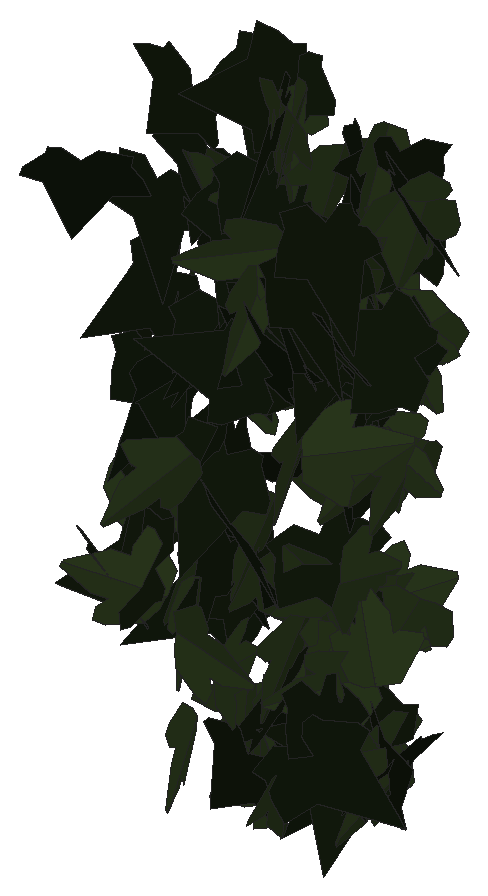
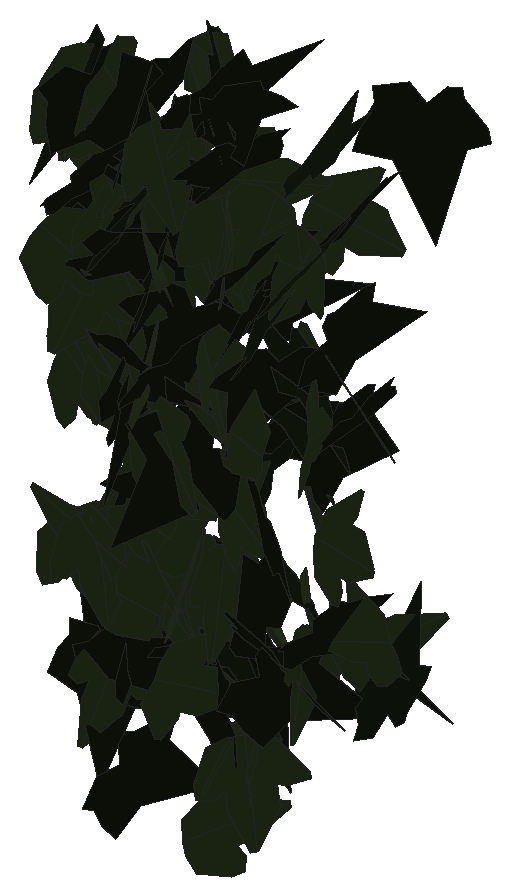
# SketchUp Ruby script. Lengths in inches.
U = 1.inch
M = Sketchup.active_model
def pt(a) = Geom::Point3d.new(a.map { |v| v * U })
def face(e, loops, mat)
  f = e.add_face(loops[0].map { |a| pt(a) })
  loops[1..].each { |l| e.add_face(l.map { |a| pt(a) }).erase! }
  f.material = f.back_material = mat if mat
  f
end
# faces: each face lists its corners as indices into pts; further lists are holes
def faces(e, pts, list, mat = nil) = list.each { |f| face(e, (f[0].is_a?(Array) ? f : [f]).map { |l| l.map { |i| pts[i] } }, mat) }
# xy, xz, yz: faces in a plane at the given z, y or x. An outline is a flat list of corners, or four numbers for a rectangle; further outlines are holes
def ring(l) = l.size == 4 ? [[l[0], l[1]], [l[2], l[1]], [l[2], l[3]], [l[0], l[3]]] : l.each_slice(2).to_a
def flat(e, list, mat, &to3) = list.each { |f| face(e, (f[0].is_a?(Array) ? f : [f]).map { |l| ring(l).map { |u, v| to3.(u, v) } }, mat) }
def xy(e, z, list, mat = nil) = flat(e, list, mat) { |x, y| [x, y, z] }
def xz(e, y, list, mat = nil) = flat(e, list, mat) { |x, z| [x, y, z] }
def yz(e, x, list, mat = nil) = flat(e, list, mat) { |y, z| [x, y, z] }
def lines(e, pts, list) = list.each { |a, b| e.add_line(pt(pts[a]), pt(pts[b])) }
# prism: a flat outline (further loops are holes) pulled along v
def prism(e, loops, v, mat = nil)
  f = face(e, loops, mat); d = Geom::Vector3d.new(v.map { |x| x * U })
  f.pushpull(f.normal.samedirection?(d) ? d.length : -d.length)
end
def box(e, o, s, mat = nil) = prism(e, [[o, [o[0] + s[0], o[1], o[2]], [o[0] + s[0], o[1] + s[1], o[2]], [o[0], o[1] + s[1], o[2]]]], [0, 0, s[2]], mat)
def at(x, y, z, deg = 0) = Geom::Transformation.translation(pt([x, y, z])) * Geom::Transformation.rotation(ORIGIN, Z_AXIS, deg.degrees)
def axes(o, x, y, z) = Geom::Transformation.new([*x, 0, *y, 0, *z, 0, *pt(o).to_a, 1])
def part(name) = M.definitions.add(name)
# library, detail: a bought-in or finely detailed component or shape, given as its bounding box
def library(name, o, s) = part(name).tap { |d| box(d.entities, o, s) }
def detail(e, o, s) = box(e.add_group.entities, o, s)
def put(e, d, t, mat = nil) = e.add_instance(d, t).tap { |i| i.material = mat if mat }
def group(e, t, mat = nil) = e.add_group.tap { |g| g.transformation = t; g.material = mat if mat }.entities
root = M.entities
M.materials.add("efeu1").color = [18, 25, 13]
M.materials.add("efeu2").color = [43, 57, 29]
c1 = part("ivyleaf_10")
p = [[0,0.5,-0.03],[-0.0625,2.02,-0.43],[-0.19,2.01,-0.46],[-0.54,1.05,-0.29],[-0.52,0.625,-0.18],[-0.83,0.76,-0.28],
  [-1.16,0.64,-0.33],[-1.15,0.33,-0.24],[-0.77,-0.39,0.02],[-0.3,-0.51,0.16],[0.04,-0.48,0.23],[-0.02,2.01,-0.4375],
  [-0.06,2.01,-0.43],[0.04,-0.49,0.23],[0.67,-0.49,0.14],[1.38,0.36,-0.2],[1.375,0.51,-0.24],[0.81,0.65,-0.19],
  [0.62,0.59,-0.15],[0.6,1.09,-0.28],[0.5,1.23,-0.31]]
faces(c1.entities,p,[[0,1,2,3,4,5,6,7,8,9,10],[11,12,0,13,14,15,16,17,18,19,20]],"efeu2")
c2 = part("ivyleaf_9")
p = [[1.54,2.16,1.25],[1.36,2.04,1.19],[-0.21,0.99,0.68],[-0.71,1.11,0.82],[-0.85,0.86,0.67],[-0.8,0.17,0.21],
  [-0.9,-0.01,0.1],[-0.67,-0.16,-0.02],[-0.08,-0.08,-0.05],[-0.03,-0.6,-0.4],[0.65,-0.88,-0.66],[0.83,-0.6,-0.49],
  [1.29,-0.42,-0.43],[1.8125,-0.07,-0.26],[1.21,0.44,0.15]]
faces(c2.entities,p,[[0,1,2,3,4,5,6,7,8,9,10,11,12,13,14]],"efeu1")
put(root,c1,axes([28.7,219.16,219.66],[-0.09561,-0.27341,0.40756],[-0.13235,-0.38548,-0.28964],[0.47259,-0.16326,0.00134]))
put(root,c1,axes([28.93,219.18,217.42],[0.02177,-0.04563,0.49744],[0.49761,0.04558,-0.0176],[-0.04374,0.49582,0.0474]))
put(root,c1,axes([28.72,219.39,216.11],[0.3565,-0.35058,0.0014],[0.00435,0.00243,-0.49998],[0.35056,0.35649,0.00478]))
put(root,c2,axes([26.43,220.35,222.25],[0.2485,0.34039,-0.26904],[-0.16173,-0.21502,-0.42144],[-0.40261,0.29647,0.00324]))
put(root,c2,axes([29.17,220.77,221.54],[0.23996,-0.43001,-0.08665],[-0.03517,0.07959,-0.49237],[0.43725,0.24239,0.00795]))
put(root,c1,axes([29.01,220.82,215.05],[0.04129,-0.48554,-0.11203],[-0.01025,0.11156,-0.48729],[0.49819,0.04254,-0.00074]))
put(root,c2,axes([29.35,220.74,215.52],[0.01382,-0.12857,-0.48299],[0.15949,0.45905,-0.11763],[0.47368,-0.15081,0.0537]))
put(root,c2,axes([29.38,221.08,222.13],[0.04971,-0.47286,-0.1547],[-0.01352,0.15413,-0.47546],[0.49734,0.05145,0.00254]))
put(root,c2,axes([28.66,221.33,220.48],[0.02304,-0.23508,0.44069],[0.13766,-0.42108,-0.23182],[0.48013,0.13201,0.04531]))
put(root,c2,axes([28.35,220.93,215.03],[0.19797,0.07499,-0.45297],[-0.42906,-0.14538,-0.21159],[-0.16344,0.47248,0.00678]))
put(root,c1,axes([27.83,221.22,215.79],[0.18255,-0.28336,-0.3693],[0.27504,-0.25438,0.33113],[-0.37554,-0.32404,0.06299]))
put(root,c2,axes([27.83,221.27,217.75],[0.22176,-0.3354,0.2972],[0.17485,-0.24055,-0.40195],[0.41261,0.2822,0.0106]))
put(root,c2,axes([27.67,221.39,218.41],[-0.23348,-0.44123,0.02835],[-0.00856,-0.02755,-0.49917],[0.44205,-0.23358,0.00531]))
put(root,c1,axes([28.17,221.4,220.74],[0.06742,0.364,-0.33609],[-0.06695,-0.32938,-0.37017],[-0.49089,0.09491,0.00433]))
put(root,c2,axes([28.18,221.36,219.68],[-0.17671,0.00384,0.46772],[-0.46563,-0.0488,-0.17552],[0.0443,-0.4976,0.02083]))
put(root,c2,axes([29.03,221.43,220.44],[0.45581,-0.17616,-0.10584],[0.10647,-0.01782,0.48821],[-0.17578,-0.4676,0.02127]))
put(root,c2,axes([29.17,221.25,215.87],[0.17957,-0.43225,-0.17583],[-0.06591,0.16301,-0.46806],[0.46196,0.19128,0.00157]))
put(root,c1,axes([28.21,221.42,221.27],[0.00952,0.09572,-0.49066],[-0.44233,-0.22704,-0.05288],[-0.23292,0.43508,0.08035]))
put(root,c2,axes([28.03,221.4375,219.92],[0.13566,-0.14789,0.45796],[0.33744,-0.31001,-0.20007],[0.34312,0.36335,0.0157]))
put(root,c1,axes([27.07,221.52,216.34],[0.35206,-0.26696,0.23406],[0.1784,-0.15198,-0.44167],[0.30696,0.39451,-0.01176]))
put(root,c2,axes([26.49,221.63,221.45],[0.0668,-0.48608,0.09622],[0.02669,-0.09342,-0.49047],[0.4948,0.07067,0.01347]))
put(root,c2,axes([28.91,221.73,220.37],[-0.0675,-0.4709,0.15395],[-0.03557,-0.15036,-0.47553],[0.49415,-0.07514,-0.0132]))
put(root,c1,axes([29.3125,221.13,219.2],[0.04861,-0.05735,-0.49432],[0.39585,0.30543,0.00349],[0.30156,-0.39169,0.07509]))
put(root,c1,axes([26.29,221.66,216.14],[0.11234,0.20323,0.44281],[-0.20859,-0.39061,0.23219],[0.44031,-0.2369,-0.00298]))
put(root,c1,axes([28.43,221.67,216.26],[0.0828,-0.41923,0.2596],[0.08923,-0.24615,-0.42597],[0.48496,0.11687,0.03406]))
put(root,c2,axes([28.5,221.39,215.68],[-0.35036,0.35599,-0.02271],[0.01212,-0.01993,-0.49946],[-0.35651,-0.35053,0.00533]))
put(root,c1,axes([28.51,221.6875,218.87],[0.15182,-0.39422,0.26747],[0.13558,-0.23336,-0.4209],[0.45669,0.20033,0.03604]))
put(root,c2,axes([26.49,221.86,218.84],[0.00288,-0.01146,-0.49986],[0.29005,-0.40712,0.011],[-0.40726,-0.29004,0.00431]))
put(root,c2,axes([29.19,221.73,215.0625],[-0.24371,-0.42591,-0.09596],[0.05035,0.08174,-0.4907],[0.43367,-0.24884,0.00305]))
put(root,c1,axes([29.64,221.91,214.77],[0.05305,-0.21525,0.44817],[0.0847,-0.44021,-0.22145],[0.48991,0.09942,-0.01025]))
put(root,c2,axes([26.45,221.96,220.11],[0.03464,-0.19944,-0.45719],[0.17323,-0.42496,0.1985],[-0.46775,-0.17215,0.03966]))
put(root,c2,axes([29.99,221.8,220.375],[-0.19617,-0.38502,-0.25155],[-0.10744,-0.22754,0.43207],[-0.44718,0.22357,0.00654]))
put(root,c1,axes([29.1875,221.76,215.9],[0.10859,0.12482,-0.47183],[-0.42786,-0.20822,-0.15355],[-0.23482,0.43711,0.06159]))
put(root,c2,axes([27.6,221.47,218.83],[-0.29344,0.3813,0.13603],[-0.09638,0.09738,-0.48086],[-0.3932,-0.30843,0.01635]))
put(root,c1,axes([27.83,221.89,217.54],[0.09572,-0.39286,0.29411],[0.11191,-0.27428,-0.4028],[0.47782,0.14294,0.03543]))
put(root,c2,axes([27.55,221.35,216.66],[-0.36639,0.1511,-0.30484],[-0.28153,0.11692,0.39632],[0.19105,0.46206,-0.0006]))
put(root,c2,axes([26.3125,221.78,219.11],[0.13386,-0.47422,-0.08485],[-0.02656,0.08067,-0.49273],[0.48102,0.13642,-0.00359]))
put(root,c2,axes([28.12,221.85,222.93],[-0.32825,0.1441,-0.34855],[0.31496,-0.14948,-0.35841],[-0.2075,-0.45485,0.00736]))
put(root,c2,axes([27.7,222.12,219.73],[-0.05327,-0.274,0.41483],[-0.05708,-0.41108,-0.27885],[0.49387,-0.07707,0.01252]))
put(root,c2,axes([29.49,221.95,214.75],[0.00895,-0.0143,0.49972],[0.21171,-0.45266,-0.01674],[0.45288,0.21189,-0.00205]))
put(root,c2,axes([25.64,221.99,215.875],[0.39691,-0.29632,-0.06822],[0.06323,-0.02929,0.49512],[-0.29742,-0.40167,0.01422]))
put(root,c1,axes([28.77,221.97,216.83],[-0.32371,-0.2417,-0.29461],[-0.18714,-0.2359,0.39916],[-0.33196,0.36869,0.06226]))
put(root,c2,axes([27.24,221.65,219.57],[-0.30711,0.39418,-0.01749],[0.00713,-0.01661,-0.49967],[-0.3945,-0.30716,0.00458]))
put(root,c1,axes([29.4375,222.05,218.77],[-0.06073,-0.28881,0.40361],[-0.06338,-0.39877,-0.29489],[0.49223,-0.08698,0.01183]))
put(root,c2,axes([26.34,221.72,216.39],[-0.4031,0.19572,0.22183],[-0.20034,0.09527,-0.44809],[-0.21766,-0.45013,0.00162]))
put(root,c1,axes([29.58,221.68,216.33],[0.46188,0.08604,0.17106],[-0.1747,0.00652,0.46844],[0.07838,-0.4925,0.03608]))
put(root,c2,axes([29.43,222.04,215],[-0.16198,-0.0601,0.4692],[-0.44629,-0.14498,-0.17264],[0.1568,-0.47473,-0.00667]))
put(root,c1,axes([28.48,222.02,215.85],[-0.02745,-0.02721,-0.4985],[0.34193,-0.3648,0.00108],[-0.36377,-0.34085,0.03864]))
put(root,c2,axes([28.875,222.1,221.06],[-0.06918,-0.49248,0.05179],[-0.00655,-0.05138,-0.49731],[0.49515,-0.06949,0.00066]))
put(root,c1,axes([29.37,221.51,217.42],[0.00592,-0.16458,-0.4721],[0.08451,0.46567,-0.16128],[0.49277,-0.07789,0.03333]))
put(root,c1,axes([28.23,221.76,222.89],[-0.41938,0.17149,0.21145],[-0.21268,0.03606,-0.45107],[-0.16996,-0.46829,0.0427]))
put(root,c2,axes([28.71,221.85,217.54],[-0.00447,-0.33806,-0.36837],[0.1627,0.34735,-0.32075],[0.47277,-0.12274,0.1069]))
put(root,c2,axes([26.45,222.29,222.35],[-0.16905,-0.27839,0.37937],[0.0698,-0.41348,-0.27232],[0.46535,-0.03911,0.17866]))
put(root,c1,axes([29.08,222.08,221.03],[-0.27917,0.04649,0.41219],[0.38525,-0.15513,0.27842],[0.15377,0.47305,0.0508]))
put(root,c2,axes([27.78,221.93,221.96],[0.09967,-0.41651,-0.25805],[0.04083,0.26948,-0.41918],[0.48826,0.06249,0.08773]))
put(root,c2,axes([29.09,222.34,218.49],[-0.03945,-0.06495,0.49419],[-0.20888,-0.44795,-0.07555],[0.45256,-0.21241,0.00821]))
put(root,c2,axes([27.1875,222.2,216.48],[0.10771,-0.1414,0.46734],[0.26087,-0.38787,-0.17748],[0.41273,0.28207,-0.00978]))
put(root,c2,axes([29.72,221.7,214.94],[-0.00003,0.49366,0.0794],[0.00006,0.0794,-0.49366],[-0.5,-0.00002,-0.00006]))
put(root,c2,axes([29.28,222,220.88],[-0.42094,-0.16819,-0.21099],[-0.19552,-0.07932,0.4533],[-0.18595,0.46413,0.001]))
put(root,c1,axes([29.72,222.24,218.78],[-0.05701,-0.43012,0.24848],[-0.03046,-0.24662,-0.43388],[0.4958,-0.06461,0.00192]))
put(root,c2,axes([27.73,222.2,215.18],[0.08788,-0.09066,-0.4838],[0.49222,0.01582,0.08644],[-0.00037,-0.49146,0.09203]))
put(root,c1,axes([29.91,222.12,222.02],[-0.2324,-0.42962,0.10682],[-0.05008,-0.09436,-0.48846],[0.43986,-0.23774,0.00083]))
put(root,c1,axes([28.12,222.125,222.79],[0.29529,-0.402,0.03463],[0.02031,-0.02806,-0.4988],[0.40298,0.29599,-0.00024]))
put(root,c1,axes([27.35,222.25,214.61],[-0.06215,-0.03309,0.49502],[0.44692,-0.22034,0.04138],[0.21541,0.44761,0.05697]))
put(root,c2,axes([27.72,222.4,222.71],[-0.16142,-0.08671,0.46522],[-0.30485,-0.3569,-0.1723],[0.36195,-0.33927,0.06235]))
put(root,c1,axes([29.8125,221.94,222.27],[-0.23008,-0.41036,-0.16932],[0.08377,0.14715,-0.47046],[0.43594,-0.24485,0.00104]))
put(root,c2,axes([29.6,222.13,219.93],[0.00117,0.0296,0.49912],[-0.48931,0.10272,-0.00494],[-0.10284,-0.48844,0.02921]))
put(root,c1,axes([27.61,222.11,214.875],[-0.0839,0.47089,-0.14568],[0.02037,-0.14434,-0.47828],[-0.49249,-0.08619,0.00503]))
put(root,c1,axes([29.36,222.42,220.54],[-0.0501,0.13372,0.47918],[0.03554,-0.47941,0.1375],[0.49621,0.04784,0.03853]))
put(root,c2,axes([25.94,222.3,219.81],[-0.34755,-0.06335,-0.35383],[0.35917,-0.08112,-0.33826],[-0.01455,-0.48929,0.10189]))
put(root,c1,axes([29.43,222.25,218.79],[-0.0869,-0.05418,-0.4894],[0.41658,-0.27304,-0.04374],[-0.26251,-0.41535,0.0926]))
put(root,c2,axes([28.55,222.41,220.37],[0.23218,-0.18571,-0.402],[0.36373,-0.17892,0.29273],[-0.25258,-0.42837,0.05201]))
put(root,c1,axes([29.42,221.92,215.14],[-0.18699,-0.38251,-0.26215],[0.1,0.24275,-0.42553],[0.45281,-0.21157,-0.01428]))
put(root,c1,axes([29.31,222.06,221.81],[-0.29787,-0.38985,-0.09641],[0.05484,0.07942,-0.4906],[0.39783,-0.30284,-0.00456]))
put(root,c1,axes([27.84,222.05,216.85],[-0.07123,-0.46881,-0.15856],[0.04694,0.15307,-0.47367],[0.49267,-0.08237,0.02221]))
put(root,c2,axes([28.34,222.03,219.84],[-0.04685,-0.23935,-0.43648],[0.1648,0.40623,-0.24045],[0.46973,-0.16639,0.04082]))
put(root,c2,axes([27.19,222.46,220.99],[-0.11546,-0.47738,0.09368],[-0.00818,-0.09436,-0.49095],[0.48642,-0.1149,0.01398]))
put(root,c1,axes([28.64,222.3,220.81],[0.23225,-0.42777,0.11434],[0.05386,-0.10086,-0.48675],[0.4395,0.23841,-0.00077]))
put(root,c1,axes([27.73,222.5,213.79],[0.00324,0.08649,0.49245],[-0.0841,-0.48535,0.08579],[0.49287,-0.08338,0.0114]))
put(root,c1,axes([27.48,222.45,221.11],[-0.09185,0.19167,-0.45258],[0.124,-0.43648,-0.21002],[-0.47559,-0.15082,0.03265]))
put(root,c1,axes([29.23,222.34,222.58],[-0.00142,0.41474,-0.27926],[-0.06058,-0.27735,-0.41159],[-0.49631,0.03267,0.05104]))
put(root,c1,axes([27.93,222.25,222.63],[-0.04796,0.47854,-0.13674],[0.01536,-0.13588,-0.48094],[-0.49746,-0.05034,-0.00167]))
put(root,c2,axes([29.625,222.1,222.37],[0.41683,-0.16053,-0.22468],[-0.20517,0.09223,-0.44654],[0.18481,0.46446,0.01101]))
put(root,c1,axes([29.66,222.3,216.76],[-0.36128,-0.26089,0.22674],[-0.18665,-0.1288,-0.44561],[0.29092,-0.40663,-0.00433]))
put(root,c2,axes([26.9,222.54,216.04],[-0.02314,-0.04708,-0.49724],[-0.08554,-0.49005,0.05038],[-0.49209,0.0874,0.01462]))
put(root,c2,axes([28.9,222.41,220.99],[0.25051,-0.41543,0.12109],[0.06616,-0.10151,-0.4851],[0.42763,0.25907,0.00411]))
put(root,c2,axes([29.0625,221.99,218.73],[0.13186,-0.11039,-0.4695],[-0.37795,0.27871,-0.17168],[0.29961,0.40017,-0.00995]))
put(root,c1,axes([27.82,222.39,220.75],[-0.22267,0.00437,0.44766],[0.43208,-0.12874,0.21618],[0.11716,0.48312,0.05355]))
put(root,c2,axes([26.88,222.54,220.36],[0.13536,-0.42557,0.22487],[0.04983,-0.21994,-0.44625],[0.47874,0.14322,-0.01713]))
put(root,c1,axes([28.34,222.2,216.26],[-0.20267,0.45533,-0.03998],[-0.03745,0.02704,0.49786],[0.45555,0.20479,0.02315]))
put(root,c2,axes([28.7,222.6,222.14],[0.16962,-0.13236,-0.45134],[0.39625,-0.21828,0.21293],[-0.2534,-0.42993,0.03085]))
put(root,c1,axes([26.62,222.16,216.33],[0.05023,-0.43839,-0.23514],[0.01717,0.23772,-0.43954],[0.49717,0.03608,0.03893]))
put(root,c2,axes([29.14,222.58,220.49],[-0.39903,-0.18804,0.2354],[-0.20175,-0.12339,-0.44054],[0.22377,-0.44656,0.0226]))
put(root,c2,axes([26.96,222.25,219.75],[-0.03191,-0.36688,-0.3382],[0.02703,0.33713,-0.36826],[0.49825,-0.04179,-0.00168]))
put(root,c1,axes([28.84,222.23,216.14],[-0.13773,-0.0462,0.47843],[0.44666,0.17154,0.14515],[-0.17755,0.46737,-0.00598]))
put(root,c1,axes([27.13,222.25,221.55],[-0.48969,0.06706,-0.07553],[0.07487,-0.00998,-0.49426],[-0.0678,-0.49538,-0.00027]))
put(root,c2,axes([29.36,222.4,222.49],[-0.01131,0.31651,-0.3869],[-0.01923,-0.38699,-0.31602],[-0.4995,0.00773,0.02093]))
put(root,c1,axes([29.35,222.36,216.89],[-0.29545,-0.4002,0.05047],[-0.02685,-0.0429,-0.49743],[0.40248,-0.29664,0.00386]))
put(root,c1,axes([27.61,222.36,221.35],[-0.36496,-0.31961,0.12105],[-0.09451,-0.07581,-0.4851],[0.32844,-0.37697,-0.00508]))
put(root,c1,axes([29.21,222.33,219.8],[-0.45007,-0.09969,0.19364],[-0.18111,-0.07562,-0.45987],[0.12097,-0.48409,0.03196]))
put(root,c2,axes([26.94,222.48,217.96],[-0.24999,0.01679,-0.43269],[0.43096,-0.03904,-0.25051],[-0.0422,-0.49819,0.00505]))
put(root,c1,axes([28.14,222.6,215.61],[0.08593,0.22943,-0.43586],[-0.25012,-0.36083,-0.23925],[-0.42433,0.25915,0.05276]))
put(root,c1,axes([27.34,222.34,214.8],[-0.41172,-0.26808,0.09281],[-0.07915,-0.04853,-0.4913],[0.27243,-0.41926,-0.00248]))
put(root,c2,axes([27.57,222.57,222.92],[-0.26661,-0.41074,-0.10103],[0.05546,0.08445,-0.48969],[0.41934,-0.27232,0.00053]))
put(root,c2,axes([27.29,222.375,216.35],[-0.43823,0.19731,0.13792],[-0.1317,0.04327,-0.4804],[-0.20151,-0.45738,0.01405]))
put(root,c2,axes([29.03,222.28,219.02],[-0.2366,0.21757,0.38299],[-0.35336,0.16581,-0.31248],[-0.26298,-0.41853,0.0753]))
put(root,c1,axes([29.74,222.56,220.42],[-0.23567,-0.21779,0.38344],[-0.26209,-0.28047,-0.32038],[0.35464,-0.352,0.01804]))
put(root,c2,axes([26.04,222.73,217],[-0.22526,-0.40694,0.18347],[-0.08867,-0.16062,-0.46512],[0.43749,-0.24209,0.00019]))
put(root,c2,axes([28.16,222.6,219.5],[-0.02988,-0.49893,-0.01326],[0.00092,0.01323,-0.49982],[0.49911,-0.02989,0.00013]))
put(root,c1,axes([26.53,222.37,221.3],[-0.44272,0.16567,-0.16296],[0.1408,-0.08769,-0.47168],[-0.18487,-0.46353,0.03099]))
put(root,c2,axes([28.67,222.75,214.43],[-0.01246,-0.02771,-0.49908],[0.15976,-0.47327,0.02229],[-0.47363,-0.15891,0.02065]))
put(root,c1,axes([28.58,222.35,217.85],[0.00321,0.01991,0.49959],[-0.49973,-0.01601,0.00385],[0.01615,-0.49935,0.0198]))
put(root,c1,axes([29.26,222.4,216.74],[0.24667,-0.06897,-0.42941],[0.42629,-0.05948,0.25444],[-0.08618,-0.49164,0.02946]))
put(root,c1,axes([25.84,222.74,218.14],[0.0754,-0.30891,0.38586],[0.12197,-0.36663,-0.31735],[0.479,0.14198,0.02007]))
put(root,c2,axes([29.29,222.82,221.45],[-0.18124,-0.38231,0.26644],[-0.0693,-0.26059,-0.42106],[0.46081,-0.18955,0.04147]))
put(root,c1,axes([28.41,222.51,222.07],[-0.14032,-0.47484,0.06957],[-0.0276,-0.06438,-0.49507],[0.47911,-0.14278,-0.00814]))
put(root,c1,axes([28.65,222.5,218.85],[-0.28502,0.38896,0.13219],[0.07912,-0.1059,0.48221],[0.40312,0.2958,-0.00119]))
put(root,c1,axes([27.19,222.45,218.8],[-0.11615,0.00014,0.48632],[0.48415,0.04723,0.11562],[-0.0459,0.49776,-0.0111]))
put(root,c1,axes([27.66,222.5,219.69],[0.13073,-0.4825,-0.01011],[-0.00019,0.01043,-0.49989],[0.48261,0.13071,0.00254]))
put(root,c1,axes([28.55,222.37,218.4375],[-0.30196,0.02248,0.39789],[-0.39749,0.01894,-0.30273],[-0.02868,-0.49914,0.00643]))
put(root,c1,axes([25.41,222.46,216.99],[0.17028,0.01647,0.46982],[0.46725,0.04908,-0.17107],[-0.05175,0.49731,0.00132]))
put(root,c2,axes([28.01,222.15,218.28],[0.39081,0.28788,0.11996],[0.09107,0.0786,-0.48531],[-0.29828,0.40118,0.009]))
put(root,c2,axes([26.27,222.8,221.28],[-0.00943,-0.42553,0.26236],[0.0674,-0.26109,-0.42106],[0.49535,0.02742,0.06229]))
put(root,c1,axes([26.12,222.76,219.39],[-0.0649,0.19708,-0.45491],[0.08479,-0.44762,-0.20602],[-0.48847,-0.10389,0.02468]))
put(root,c1,axes([29.41,222.39,220.09],[-0.45039,-0.14428,-0.16228],[0.15559,0.04622,-0.47292],[0.15147,-0.4765,0.00326]))
